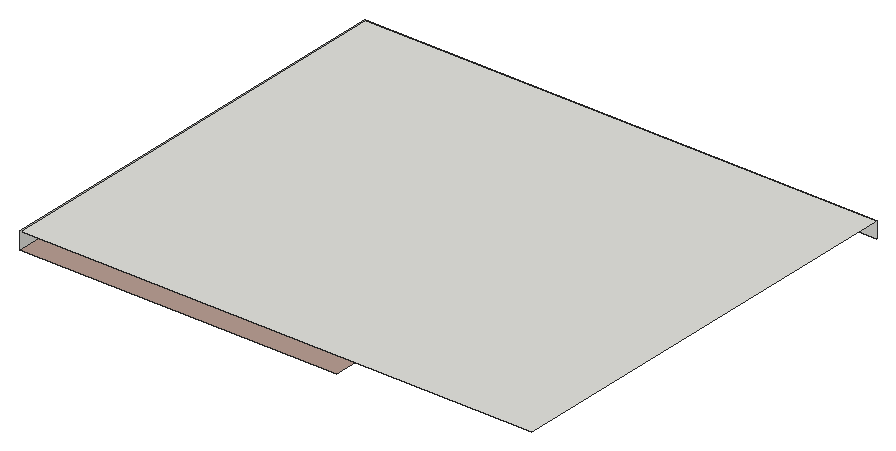
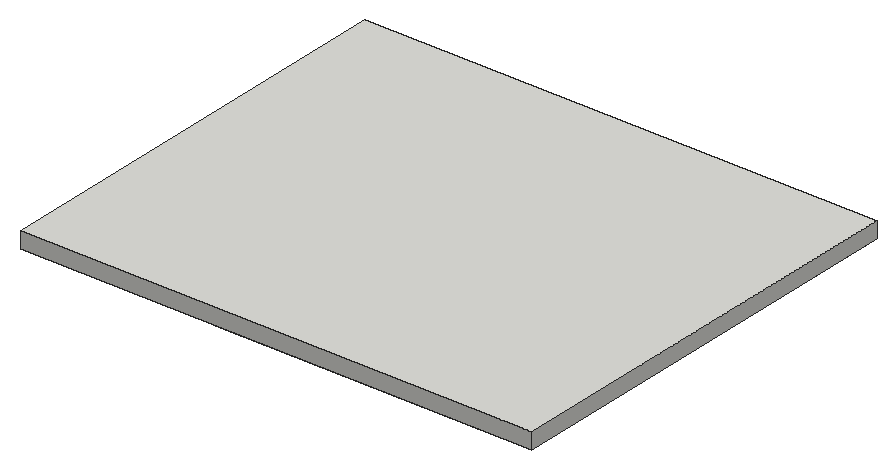
# SketchUp Ruby script. Lengths in inches.
U = 1.inch
M = Sketchup.active_model
def pt(a) = Geom::Point3d.new(a.map { |v| v * U })
def face(e, loops, mat)
  f = e.add_face(loops[0].map { |a| pt(a) })
  loops[1..].each { |l| e.add_face(l.map { |a| pt(a) }).erase! }
  f.material = f.back_material = mat if mat
  f
end
# faces: each face lists its corners as indices into pts; further lists are holes
def faces(e, pts, list, mat = nil) = list.each { |f| face(e, (f[0].is_a?(Array) ? f : [f]).map { |l| l.map { |i| pts[i] } }, mat) }
# xy, xz, yz: faces in a plane at the given z, y or x. An outline is a flat list of corners, or four numbers for a rectangle; further outlines are holes
def ring(l) = l.size == 4 ? [[l[0], l[1]], [l[2], l[1]], [l[2], l[3]], [l[0], l[3]]] : l.each_slice(2).to_a
def flat(e, list, mat, &to3) = list.each { |f| face(e, (f[0].is_a?(Array) ? f : [f]).map { |l| ring(l).map { |u, v| to3.(u, v) } }, mat) }
def xy(e, z, list, mat = nil) = flat(e, list, mat) { |x, y| [x, y, z] }
def xz(e, y, list, mat = nil) = flat(e, list, mat) { |x, z| [x, y, z] }
def yz(e, x, list, mat = nil) = flat(e, list, mat) { |y, z| [x, y, z] }
def lines(e, pts, list) = list.each { |a, b| e.add_line(pt(pts[a]), pt(pts[b])) }
# prism: a flat outline (further loops are holes) pulled along v
def prism(e, loops, v, mat = nil)
  f = face(e, loops, mat); d = Geom::Vector3d.new(v.map { |x| x * U })
  f.pushpull(f.normal.samedirection?(d) ? d.length : -d.length)
end
def box(e, o, s, mat = nil) = prism(e, [[o, [o[0] + s[0], o[1], o[2]], [o[0] + s[0], o[1] + s[1], o[2]], [o[0], o[1] + s[1], o[2]]]], [0, 0, s[2]], mat)
def at(x, y, z, deg = 0) = Geom::Transformation.translation(pt([x, y, z])) * Geom::Transformation.rotation(ORIGIN, Z_AXIS, deg.degrees)
def axes(o, x, y, z) = Geom::Transformation.new([*x, 0, *y, 0, *z, 0, *pt(o).to_a, 1])
def part(name) = M.definitions.add(name)
# library, detail: a bought-in or finely detailed component or shape, given as its bounding box
def library(name, o, s) = part(name).tap { |d| box(d.entities, o, s) }
def detail(e, o, s) = box(e.add_group.entities, o, s)
def put(e, d, t, mat = nil) = e.add_instance(d, t).tap { |i| i.material = mat if mat }
def group(e, t, mat = nil) = e.add_group.tap { |g| g.transformation = t; g.material = mat if mat }.entities
root = M.entities
M.materials.add("Emissive").color = [229, 220, 142]
M.materials.add("Emissive\#1").color = [244, 244, 244]
M.materials.add("PDM_Metal_01").color = [44, 44, 42]
M.materials.add("[Color A01]2").color = [191, 160, 139]
M.materials.add("[Color A01]3").color = [183, 157, 146]
c1 = library("Group\#200",[0,0,0],[4.97,5,2.25])
c2 = library("Component\#2",[0,0,0],[16.18,4.625,1.6875])
box(root,[133.1875,41.59,119.4375],[5.94,56.86,4],"PDM_Metal_01")
xy(root,125.75,[[[44.35,127.46,43.23,127.72,42.22,128.26,41.38,129.05,40.77,130.02,40.4375,131.125,40.4,132.27,40.66,133.39,41.2,134.41,41.99,135.25,42.96,135.85,44.0625,136.1875,45.21,136.23,46.33,135.97,47.35,135.42,48.1875,134.64,48.79,133.66,49.13,132.5625,49.17,131.41,48.91,130.29,48.36,129.28,47.58,128.4375,46.6,127.83,45.5,127.5],[44.41,128.05,45.4,128.08,46.36,128.37,47.2,128.9,47.88,129.62,48.35,130.5,48.58,131.47,48.54,132.46,48.26,133.42,47.73,134.26,47,134.94,46.125,135.41,45.16,135.64,44.16,135.6,43.21,135.31,42.36,134.79,41.68,134.0625,41.21,133.18,40.99,132.22,41.02,131.22,41.31,130.27,41.84,129.42,42.5625,128.74,43.44,128.27]],[[89.16,127.46,88.04,127.72,87.03,128.26,86.1875,129.05,85.58,130.02,85.25,131.125,85.21,132.27,85.47,133.39,86.01,134.41,86.8,135.25,87.77,135.85,88.875,136.1875,90.02,136.23,91.14,135.97,92.16,135.42,93,134.64,93.6,133.66,93.9375,132.5625,93.98,131.41,93.72,130.29,93.17,129.28,92.39,128.4375,91.41,127.83,90.3125,127.5],[89.22,128.05,90.21,128.08,91.17,128.37,92.01,128.9,92.69,129.62,93.16,130.5,93.39,131.47,93.35,132.46,93.06,133.42,92.54,134.26,91.8125,134.94,90.93,135.41,89.97,135.64,88.97,135.6,88.02,135.31,87.17,134.79,86.49,134.0625,86.02,133.18,85.8,132.22,85.83,131.22,86.12,130.27,86.65,129.42,87.37,128.74,88.25,128.27]]])
xy(root,126,[[[44.41,128.05,43.44,128.27,42.5625,128.74,41.84,129.42,41.31,130.27,41.02,131.22,40.99,132.22,41.21,133.18,41.68,134.0625,42.36,134.79,43.21,135.31,44.16,135.6,45.16,135.64,46.125,135.41,47,134.94,47.73,134.26,48.26,133.42,48.54,132.46,48.58,131.47,48.35,130.5,47.88,129.62,47.2,128.9,46.36,128.37,45.4,128.08],[44.46,128.53,45.33,128.56,46.16,128.81,46.9,129.27,47.49,129.9,47.9,130.67,48.1,131.52,48.07,132.39,47.82,133.22,47.36,133.96,46.72,134.55,45.96,134.96,45.11,135.16,44.24,135.13,43.41,134.875,42.67,134.42,42.08,133.78,41.67,133.01,41.47,132.17,41.5,131.3,41.75,130.47,42.21,129.73,42.84,129.14,43.61,128.73]],[[89.22,128.05,88.25,128.27,87.37,128.74,86.65,129.42,86.12,130.27,85.83,131.22,85.8,132.22,86.02,133.18,86.49,134.0625,87.17,134.79,88.02,135.31,88.97,135.6,89.97,135.64,90.93,135.41,91.8125,134.94,92.54,134.26,93.06,133.42,93.35,132.46,93.39,131.47,93.16,130.5,92.69,129.62,92.01,128.9,91.17,128.37,90.21,128.08],[89.27,128.53,90.14,128.56,90.97,128.81,91.71,129.27,92.3,129.9,92.71,130.67,92.91,131.52,92.88,132.39,92.625,133.22,92.17,133.96,91.53,134.55,90.76,134.96,89.92,135.16,89.05,135.13,88.22,134.875,87.48,134.42,86.89,133.78,86.48,133.01,86.28,132.17,86.31,131.3,86.56,130.47,87.02,129.73,87.65,129.14,88.42,128.73]]],"Emissive\#1")
xy(root,126,[[[34.78,43.66,99.59,141.84],[44.35,127.46,43.23,127.72,42.22,128.26,41.38,129.05,40.77,130.02,40.4375,131.125,40.4,132.27,40.66,133.39,41.2,134.41,41.99,135.25,42.96,135.85,44.0625,136.1875,45.21,136.23,46.33,135.97,47.35,135.42,48.1875,134.64,48.79,133.66,49.13,132.5625,49.17,131.41,48.91,130.29,48.36,129.28,47.58,128.4375,46.6,127.83,45.5,127.5],[89.16,127.46,88.04,127.72,87.03,128.26,86.1875,129.05,85.58,130.02,85.25,131.125,85.21,132.27,85.47,133.39,86.01,134.41,86.8,135.25,87.77,135.85,88.875,136.1875,90.02,136.23,91.14,135.97,92.16,135.42,93,134.64,93.6,133.66,93.9375,132.5625,93.98,131.41,93.72,130.29,93.17,129.28,92.39,128.4375,91.41,127.83,90.3125,127.5],[89.16,49.27,88.04,49.53,87.03,50.08,86.1875,50.86,85.58,51.84,85.25,52.9375,85.21,54.09,85.47,55.21,86.01,56.22,86.8,57.0625,87.77,57.67,88.875,58,90.02,58.04,91.14,57.78,92.16,57.24,93,56.45,93.6,55.48,93.9375,54.375,93.98,53.23,93.72,52.11,93.17,51.09,92.39,50.25,91.41,49.65,90.3125,49.3125],[44.35,49.27,43.23,49.53,42.22,50.08,41.38,50.86,40.77,51.84,40.4375,52.9375,40.4,54.09,40.66,55.21,41.2,56.22,41.99,57.0625,42.96,57.67,44.0625,58,45.21,58.04,46.33,57.78,47.35,57.24,48.1875,56.45,48.79,55.48,49.13,54.375,49.17,53.23,48.91,52.11,48.36,51.09,47.58,50.25,46.6,49.65,45.5,49.3125]],[[44.35,127.46,45.5,127.5,46.6,127.83,47.58,128.4375,48.36,129.28,48.91,130.29,49.17,131.41,49.13,132.5625,48.79,133.66,48.1875,134.64,47.35,135.42,46.33,135.97,45.21,136.23,44.0625,136.1875,42.96,135.85,41.99,135.25,41.2,134.41,40.66,133.39,40.4,132.27,40.4375,131.125,40.77,130.02,41.38,129.05,42.22,128.26,43.23,127.72],[44.41,128.05,43.44,128.27,42.5625,128.74,41.84,129.42,41.31,130.27,41.02,131.22,40.99,132.22,41.21,133.18,41.68,134.0625,42.36,134.79,43.21,135.31,44.16,135.6,45.16,135.64,46.125,135.41,47,134.94,47.73,134.26,48.26,133.42,48.54,132.46,48.58,131.47,48.35,130.5,47.88,129.62,47.2,128.9,46.36,128.37,45.4,128.08]],[[89.16,127.46,90.3125,127.5,91.41,127.83,92.39,128.4375,93.17,129.28,93.72,130.29,93.98,131.41,93.9375,132.5625,93.6,133.66,93,134.64,92.16,135.42,91.14,135.97,90.02,136.23,88.875,136.1875,87.77,135.85,86.8,135.25,86.01,134.41,85.47,133.39,85.21,132.27,85.25,131.125,85.58,130.02,86.1875,129.05,87.03,128.26,88.04,127.72],[89.22,128.05,88.25,128.27,87.37,128.74,86.65,129.42,86.12,130.27,85.83,131.22,85.8,132.22,86.02,133.18,86.49,134.0625,87.17,134.79,88.02,135.31,88.97,135.6,89.97,135.64,90.93,135.41,91.8125,134.94,92.54,134.26,93.06,133.42,93.35,132.46,93.39,131.47,93.16,130.5,92.69,129.62,92.01,128.9,91.17,128.37,90.21,128.08]]],"[Color A01]2")
xy(root,126,[[[9,9,125.375,167.625],[19.48,28.36,114.89,157.14]]],"[Color A01]3")
xy(root,126.375,[[44.46,128.53,43.61,128.73,42.84,129.14,42.21,129.73,41.75,130.47,41.5,131.3,41.47,132.17,41.67,133.01,42.08,133.78,42.67,134.42,43.41,134.875,44.24,135.13,45.11,135.16,45.96,134.96,46.72,134.55,47.36,133.96,47.82,133.22,48.07,132.39,48.1,131.52,47.9,130.67,47.49,129.9,46.9,129.27,46.16,128.81,45.33,128.56],[89.27,128.53,88.42,128.73,87.65,129.14,87.02,129.73,86.56,130.47,86.31,131.3,86.28,132.17,86.48,133.01,86.89,133.78,87.48,134.42,88.22,134.875,89.05,135.13,89.92,135.16,90.76,134.96,91.53,134.55,92.17,133.96,92.625,133.22,92.88,132.39,92.91,131.52,92.71,130.67,92.3,129.9,91.71,129.27,90.97,128.81,90.14,128.56]],"Emissive\#1")
xy(root,128.22,[[18.79,28.36,19.48,157.83],[114.89,28.36,115.58,157.83],[19.48,157.14,114.89,157.83]])
xy(root,128.6875,[[34.78,43.66,35.66,140.97],[98.72,43.66,99.59,140.97],[34.78,140.97,99.59,141.84]])
xy(root,130.4375,[[[18.79,27.67,115.58,157.83],[35.66,44.53,98.72,140.97]]],"[Color A01]3")
xy(root,132,[[9,9,197.1875,167.625]])
xz(root,140.97,[[35.66,128.6875,98.72,130.4375]],"Emissive")
xz(root,141.84,[[34.78,126,99.59,128.6875]])
xz(root,157.14,[[19.48,126,114.89,128.22]])
xz(root,157.83,[[18.79,128.22,115.58,130.4375]],"Emissive")
xz(root,167.625,[[9,126,197.1875,132]])
yz(root,9,[[9,126,167.625,132]])
yz(root,18.79,[[27.67,128.22,157.83,130.4375]],"Emissive")
yz(root,19.48,[[28.36,126,157.14,128.22]])
yz(root,34.78,[[43.66,126,141.84,128.6875]])
yz(root,35.66,[[44.53,128.6875,140.97,130.4375]],"Emissive")
yz(root,98.72,[[44.53,128.6875,140.97,130.4375]],"Emissive")
yz(root,99.59,[[43.66,126,141.84,128.6875]])
yz(root,114.89,[[28.36,126,157.14,128.22]])
yz(root,115.58,[[27.67,128.22,157.83,130.4375]],"Emissive")
p = [[41.2,56.22,126],[41.99,57.0625,126],[41.99,57.0625,125.75],[41.2,56.22,125.75],[86.01,56.22,126],[86.8,57.0625,126],
  [86.8,57.0625,125.75],[86.01,56.22,125.75],[47.35,57.24,126],[48.1875,56.45,126],[48.1875,56.45,125.75],[47.35,57.24,125.75],
  [92.16,57.24,126],[93,56.45,126],[93,56.45,125.75],[92.16,57.24,125.75],[43.21,57.13,126],[42.36,56.6,126],
  [42.36,56.6,125.75],[43.21,57.13,125.75],[88.02,57.13,126],[87.17,56.6,126],[87.17,56.6,125.75],[88.02,57.13,125.75],
  [47,56.76,126],[46.125,57.23,126],[46.125,57.23,125.75],[47,56.76,125.75],[91.8125,56.76,126],[90.93,57.23,126],
  [90.93,57.23,125.75],[91.8125,56.76,125.75],[42.96,57.67,126],[42.96,57.67,125.75],[44.16,57.42,126],[44.16,57.42,125.75],
  [87.77,57.67,126],[87.77,57.67,125.75],[88.97,57.42,126],[88.97,57.42,125.75],[45.16,57.45,126],[45.16,57.45,125.75],
  [46.33,57.78,126],[46.33,57.78,125.75],[89.97,57.45,126],[89.97,57.45,125.75],[91.14,57.78,126],[91.14,57.78,125.75],
  [44.0625,58,126],[44.0625,58,125.75],[88.875,58,126],[88.875,58,125.75],[45.21,58.04,126],[45.21,58.04,125.75],
  [90.02,58.04,126],[90.02,58.04,125.75],[44.35,127.46,126],[43.23,127.72,126],[43.23,127.72,125.75],[44.35,127.46,125.75],
  [45.5,127.5,126],[45.5,127.5,125.75],[46.6,127.83,126],[46.6,127.83,125.75],[89.16,127.46,126],[88.04,127.72,126],
  [88.04,127.72,125.75],[89.16,127.46,125.75],[90.3125,127.5,126],[90.3125,127.5,125.75],[91.41,127.83,126],[91.41,127.83,125.75],
  [42.22,128.26,126],[42.22,128.26,125.75],[87.03,128.26,126],[87.03,128.26,125.75],[47.58,128.4375,126],[47.58,128.4375,125.75],
  [92.39,128.4375,126],[92.39,128.4375,125.75],[43.44,128.27,126],[44.41,128.05,126],[44.41,128.05,125.75],[43.44,128.27,125.75],
  [45.4,128.08,126],[45.4,128.08,125.75],[88.25,128.27,126],[89.22,128.05,126],[89.22,128.05,125.75],[88.25,128.27,125.75],
  [90.21,128.08,126],[90.21,128.08,125.75],[46.36,128.37,126],[46.36,128.37,125.75],[91.17,128.37,126],[91.17,128.37,125.75],
  [41.38,129.05,126],[41.38,129.05,125.75],[42.5625,128.74,126],[42.5625,128.74,125.75],[86.1875,129.05,126],[86.1875,129.05,125.75],
  [87.37,128.74,126],[87.37,128.74,125.75],[47.2,128.9,126],[47.2,128.9,125.75],[48.36,129.28,126],[48.36,129.28,125.75],
  [92.01,128.9,126],[92.01,128.9,125.75],[93.17,129.28,126],[93.17,129.28,125.75],[41.84,129.42,126],[41.84,129.42,125.75],
  [86.65,129.42,126],[86.65,129.42,125.75],[47.88,129.62,126],[47.88,129.62,125.75],[92.69,129.62,126],[92.69,129.62,125.75],
  [40.77,130.02,126],[40.77,130.02,125.75],[85.58,130.02,126],[85.58,130.02,125.75],[48.91,130.29,126],[48.91,130.29,125.75],
  [93.72,130.29,126],[93.72,130.29,125.75],[41.31,130.27,126],[41.31,130.27,125.75],[86.12,130.27,126],[86.12,130.27,125.75],
  [48.35,130.5,126],[48.35,130.5,125.75],[93.16,130.5,126],[93.16,130.5,125.75],[40.4375,131.125,126],[40.4375,131.125,125.75],
  [85.25,131.125,126],[85.25,131.125,125.75],[41.02,131.22,126],[41.02,131.22,125.75],[49.17,131.41,126],[49.17,131.41,125.75],
  [85.83,131.22,126],[85.83,131.22,125.75],[93.98,131.41,126],[93.98,131.41,125.75],[48.58,131.47,126],[48.58,131.47,125.75],
  [93.39,131.47,126],[93.39,131.47,125.75],[40.4,132.27,126],[40.4,132.27,125.75],[85.21,132.27,126],[85.21,132.27,125.75],
  [40.99,132.22,126],[40.99,132.22,125.75],[85.8,132.22,126],[85.8,132.22,125.75],[49.13,132.5625,126],[49.13,132.5625,125.75],
  [93.9375,132.5625,126],[93.9375,132.5625,125.75],[48.54,132.46,126],[48.54,132.46,125.75],[93.35,132.46,126],[93.35,132.46,125.75],
  [41.21,133.18,126],[41.21,133.18,125.75],[86.02,133.18,126],[86.02,133.18,125.75],[40.66,133.39,126],[40.66,133.39,125.75],
  [85.47,133.39,126],[85.47,133.39,125.75],[48.26,133.42,126],[48.26,133.42,125.75],[93.06,133.42,126],[93.06,133.42,125.75],
  [48.79,133.66,126],[48.79,133.66,125.75],[93.6,133.66,126],[93.6,133.66,125.75],[41.68,134.0625,126],[41.68,134.0625,125.75],
  [86.49,134.0625,126],[86.49,134.0625,125.75],[41.2,134.41,126],[41.2,134.41,125.75],[47.73,134.26,126],[47.73,134.26,125.75],
  [86.01,134.41,126],[86.01,134.41,125.75],[92.54,134.26,126],[92.54,134.26,125.75],[48.1875,134.64,126],[48.1875,134.64,125.75],
  [93,134.64,126],[93,134.64,125.75],[42.36,134.79,126],[42.36,134.79,125.75],[87.17,134.79,126],[87.17,134.79,125.75],
  [47,134.94,126],[47,134.94,125.75],[91.8125,134.94,126],[91.8125,134.94,125.75],[41.99,135.25,126],[41.99,135.25,125.75],
  [86.8,135.25,126],[86.8,135.25,125.75],[47.35,135.42,126],[47.35,135.42,125.75],[92.16,135.42,126],[92.16,135.42,125.75],
  [43.21,135.31,126],[43.21,135.31,125.75],[88.02,135.31,126],[88.02,135.31,125.75],[46.125,135.41,126],[46.125,135.41,125.75],
  [90.93,135.41,126],[90.93,135.41,125.75],[42.96,135.85,126],[42.96,135.85,125.75],[87.77,135.85,126],[87.77,135.85,125.75],
  [44.16,135.6,126],[44.16,135.6,125.75],[88.97,135.6,126],[88.97,135.6,125.75],[45.16,135.64,126],[45.16,135.64,125.75],
  [46.33,135.97,126],[46.33,135.97,125.75],[89.97,135.64,126],[89.97,135.64,125.75],[91.14,135.97,126],[91.14,135.97,125.75],
  [44.0625,136.1875,126],[44.0625,136.1875,125.75],[88.875,136.1875,126],[88.875,136.1875,125.75],[45.21,136.23,126],[45.21,136.23,125.75],
  [90.02,136.23,126],[90.02,136.23,125.75],[45.96,56.77,126],[46.72,56.36,126],[46.72,56.36,126.375],[45.96,56.77,126.375],
  [90.76,56.77,126],[91.53,56.36,126],[91.53,56.36,126.375],[90.76,56.77,126.375],[43.41,56.69,126],[44.24,56.94,126],
  [44.24,56.94,126.375],[43.41,56.69,126.375],[88.22,56.69,126],[89.05,56.94,126],[89.05,56.94,126.375],[88.22,56.69,126.375],
  [45.11,56.97,126],[45.11,56.97,126.375],[89.92,56.97,126],[89.92,56.97,126.375],[44.46,128.53,126],[43.61,128.73,126],
  [43.61,128.73,126.375],[44.46,128.53,126.375],[45.33,128.56,126],[45.33,128.56,126.375],[89.27,128.53,126],[88.42,128.73,126],
  [88.42,128.73,126.375],[89.27,128.53,126.375],[90.14,128.56,126],[90.14,128.56,126.375],[46.16,128.81,126],[46.16,128.81,126.375],
  [90.97,128.81,126],[90.97,128.81,126.375],[42.84,129.14,126],[42.84,129.14,126.375],[87.65,129.14,126],[87.65,129.14,126.375],
  [46.9,129.27,126],[46.9,129.27,126.375],[91.71,129.27,126],[91.71,129.27,126.375],[42.21,129.73,126],[42.21,129.73,126.375],
  [87.02,129.73,126],[87.02,129.73,126.375],[47.49,129.9,126],[47.49,129.9,126.375],[92.3,129.9,126],[92.3,129.9,126.375],
  [41.75,130.47,126],[41.75,130.47,126.375],[86.56,130.47,126],[86.56,130.47,126.375],[47.9,130.67,126],[47.9,130.67,126.375],
  [92.71,130.67,126],[92.71,130.67,126.375],[41.5,131.3,126],[41.5,131.3,126.375],[86.31,131.3,126],[86.31,131.3,126.375],
  [48.1,131.52,126],[48.1,131.52,126.375],[92.91,131.52,126],[92.91,131.52,126.375],[41.47,132.17,126],[41.47,132.17,126.375],
  [86.28,132.17,126],[86.28,132.17,126.375],[48.07,132.39,126],[48.07,132.39,126.375],[92.88,132.39,126],[92.88,132.39,126.375],
  [41.67,133.01,126],[41.67,133.01,126.375],[86.48,133.01,126],[86.48,133.01,126.375],[47.82,133.22,126],[47.82,133.22,126.375],
  [92.625,133.22,126],[92.625,133.22,126.375],[42.08,133.78,126],[42.08,133.78,126.375],[86.89,133.78,126],[86.89,133.78,126.375],
  [47.36,133.96,126],[47.36,133.96,126.375],[92.17,133.96,126],[92.17,133.96,126.375],[42.67,134.42,126],[42.67,134.42,126.375],
  [87.48,134.42,126],[87.48,134.42,126.375],[46.72,134.55,126],[46.72,134.55,126.375],[91.53,134.55,126],[91.53,134.55,126.375],
  [43.41,134.875,126],[43.41,134.875,126.375],[88.22,134.875,126],[88.22,134.875,126.375],[45.96,134.96,126],[45.96,134.96,126.375],
  [90.76,134.96,126],[90.76,134.96,126.375],[44.24,135.13,126],[44.24,135.13,126.375],[89.05,135.13,126],[89.05,135.13,126.375],
  [45.11,135.16,126],[45.11,135.16,126.375],[89.92,135.16,126],[89.92,135.16,126.375]]
faces(root,p,[[0,1,2,3],[4,5,6,7],[8,9,10,11],[12,13,14,15],[16,17,18,19],[20,21,22,23],[24,25,26,27],[28,29,30,31],
  [1,32,33,2],[34,16,19,35],[5,36,37,6],[38,20,23,39],[25,40,41,26],[42,8,11,43],[29,44,45,30],[46,12,15,47],
  [40,34,35,41],[44,38,39,45],[32,48,49,33],[36,50,51,37],[52,42,43,53],[54,46,47,55],[48,52,53,49],[50,54,55,51],
  [56,57,58,59],[60,56,59,61],[62,60,61,63],[64,65,66,67],[68,64,67,69],[70,68,69,71],[57,72,73,58],[65,74,75,66],
  [76,62,63,77],[78,70,71,79],[80,81,82,83],[81,84,85,82],[86,87,88,89],[87,90,91,88],[84,92,93,85],[90,94,95,91],
  [72,96,97,73],[98,80,83,99],[74,100,101,75],[102,86,89,103],[92,104,105,93],[106,76,77,107],[94,108,109,95],[110,78,79,111],
  [112,98,99,113],[114,102,103,115],[104,116,117,105],[108,118,119,109],[96,120,121,97],[100,122,123,101],[124,106,107,125],[126,110,111,127],
  [128,112,113,129],[130,114,115,131],[116,132,133,117],[118,134,135,119],[120,136,137,121],[122,138,139,123],[140,128,129,141],[142,124,125,143],
  [144,130,131,145],[146,126,127,147],[132,148,149,133],[134,150,151,135],[136,152,153,137],[138,154,155,139],[156,140,141,157],[158,144,145,159],
  [160,142,143,161],[162,146,147,163],[148,164,165,149],[150,166,167,151],[168,156,157,169],[170,158,159,171],[152,172,173,153],[154,174,175,155],
  [164,176,177,165],[166,178,179,167],[180,160,161,181],[182,162,163,183],[184,168,169,185],[186,170,171,187],[172,188,189,173],[176,190,191,177],
  [174,192,193,175],[178,194,195,179],[196,180,181,197],[198,182,183,199],[200,184,185,201],[202,186,187,203],[190,204,205,191],[194,206,207,195],
  [188,208,209,189],[192,210,211,193],[212,196,197,213],[214,198,199,215],[216,200,201,217],[218,202,203,219],[204,220,221,205],[206,222,223,207],
  [208,224,225,209],[210,226,227,211],[228,216,217,229],[230,218,219,231],[220,232,233,221],[234,212,213,235],[222,236,237,223],[238,214,215,239],
  [232,228,229,233],[236,230,231,237],[224,240,241,225],[226,242,243,227],[244,234,235,245],[246,238,239,247],[240,244,245,241],[242,246,247,243]])
faces(root,p,[[248,249,250,251],[252,253,254,255],[256,257,258,259],[260,261,262,263],[264,248,251,265],[266,252,255,267],[257,264,265,258],[261,266,267,262],
  [268,269,270,271],[272,268,271,273],[274,275,276,277],[278,274,277,279],[280,272,273,281],[282,278,279,283],[269,284,285,270],[275,286,287,276],
  [288,280,281,289],[290,282,283,291],[284,292,293,285],[286,294,295,287],[296,288,289,297],[298,290,291,299],[292,300,301,293],[294,302,303,295],
  [304,296,297,305],[306,298,299,307],[300,308,309,301],[302,310,311,303],[312,304,305,313],[314,306,307,315],[308,316,317,309],[310,318,319,311],
  [320,312,313,321],[322,314,315,323],[316,324,325,317],[318,326,327,319],[328,320,321,329],[330,322,323,331],[324,332,333,325],[326,334,335,327],
  [336,328,329,337],[338,330,331,339],[332,340,341,333],[334,342,343,335],[344,336,337,345],[346,338,339,347],[340,348,349,341],[342,350,351,343],
  [352,344,345,353],[354,346,347,355],[348,356,357,349],[350,358,359,351],[360,352,353,361],[362,354,355,363],[356,360,361,357],[358,362,363,359]],"Emissive\#1")
put(root,c1,axes([130.91,78.71,91.86],[0,-1.3225,0],[1.3225,0,0],[0,0,1.3225]))
put(root,c2,axes([73.22,78.52,126],[-0.5,0.86603,0],[0.86603,0.5,0],[0,0,-1]))
put(root,c2,axes([57.04,80.89,126],[0.5,0.86603,0],[0.86603,-0.5,0],[0,0,-1]))
put(root,c2,axes([83.36,91.34,126],[-1,0,0],[0,1,0],[0,0,-1]))
put(root,c2,axes([51.01,96.09,126],[1,0,0],[0,-1,0],[0,0,-1]))
put(root,c2,axes([77.33,106.54,126],[-0.5,-0.86603,0],[-0.86603,0.5,0],[0,0,-1]))
put(root,c2,axes([61.16,108.91,126],[0.5,-0.86603,0],[-0.86603,-0.5,0],[0,0,-1]))
